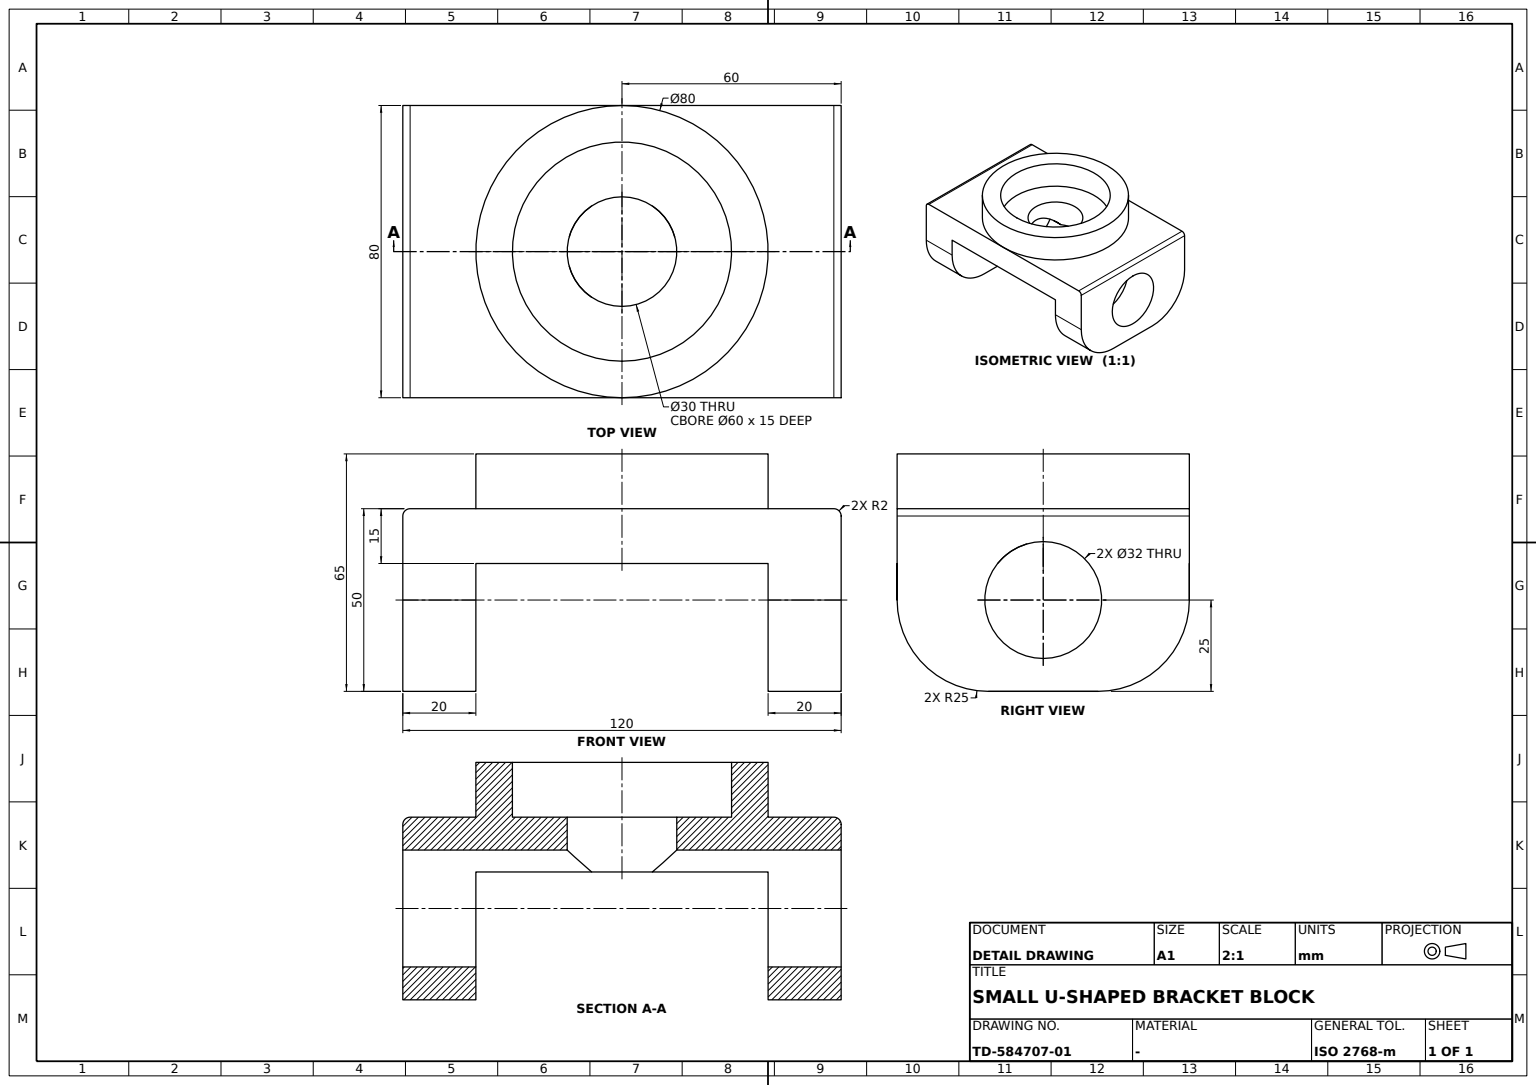
ISO-10303-21;
HEADER;
FILE_DESCRIPTION((''),'2;1');
FILE_NAME('','',(''),(''),'','','');
FILE_SCHEMA(('AUTOMOTIVE_DESIGN'));
ENDSEC;
DATA;
#1=APPLICATION_CONTEXT('');
#2=PRODUCT_CONTEXT('',#1,'mechanical');
#3=PRODUCT('','','',(#2));
#4=PRODUCT_DEFINITION_FORMATION('','',#3);
#5=PRODUCT_DEFINITION_CONTEXT('',#1,'design');
#6=PRODUCT_DEFINITION('','',#4,#5);
#7=PRODUCT_DEFINITION_SHAPE('','',#6);
#8=(LENGTH_UNIT()NAMED_UNIT(*)SI_UNIT(.MILLI.,.METRE.));
#9=(NAMED_UNIT(*)PLANE_ANGLE_UNIT()SI_UNIT($,.RADIAN.));
#10=(NAMED_UNIT(*)SI_UNIT($,.STERADIAN.)SOLID_ANGLE_UNIT());
#11=UNCERTAINTY_MEASURE_WITH_UNIT(LENGTH_MEASURE(0.005),#8,'distance_accuracy_value','');
#12=(GEOMETRIC_REPRESENTATION_CONTEXT(3)GLOBAL_UNCERTAINTY_ASSIGNED_CONTEXT((#11))GLOBAL_UNIT_ASSIGNED_CONTEXT((#8,#9,#10))REPRESENTATION_CONTEXT('',''));
#13=CARTESIAN_POINT('',(12.489996,40.,0.));
#14=VERTEX_POINT('',#13);
#15=CARTESIAN_POINT('',(40.,40.,0.));
#16=VERTEX_POINT('',#15);
#17=CARTESIAN_POINT('',(0.,40.,0.));
#18=DIRECTION('',(1.,0.,0.));
#19=VECTOR('',#18,1000.);
#20=LINE('',#17,#19);
#21=EDGE_CURVE('',#14,#16,#20,.T.);
#22=ORIENTED_EDGE('',*,*,#21,.T.);
#23=CARTESIAN_POINT('',(40.,-40.,0.));
#24=VERTEX_POINT('',#23);
#25=CARTESIAN_POINT('',(40.,0.,0.));
#26=DIRECTION('',(0.,1.,0.));
#27=VECTOR('',#26,1000.);
#28=LINE('',#25,#27);
#29=EDGE_CURVE('',#24,#16,#28,.T.);
#30=ORIENTED_EDGE('',*,*,#29,.F.);
#31=CARTESIAN_POINT('',(12.489996,-40.,0.));
#32=VERTEX_POINT('',#31);
#33=CARTESIAN_POINT('',(0.,-40.,0.));
#34=LINE('',#33,#19);
#35=EDGE_CURVE('',#32,#24,#34,.T.);
#36=ORIENTED_EDGE('',*,*,#35,.F.);
#37=CARTESIAN_POINT('',(12.489996,-8.306624,0.));
#38=VERTEX_POINT('',#37);
#39=LINE('',#31,#27);
#40=EDGE_CURVE('',#38,#32,#39,.F.);
#41=ORIENTED_EDGE('',*,*,#40,.F.);
#42=CARTESIAN_POINT('',(12.489996,8.306624,0.));
#43=VERTEX_POINT('',#42);
#44=CARTESIAN_POINT('',(0.,0.,0.));
#45=DIRECTION('',(0.,0.,-1.));
#46=DIRECTION('',(-1.,0.,0.));
#47=AXIS2_PLACEMENT_3D('',#44,#45,#46);
#48=CIRCLE('',#47,15.);
#49=EDGE_CURVE('',#38,#43,#48,.F.);
#50=ORIENTED_EDGE('',*,*,#49,.T.);
#51=LINE('',#42,#27);
#52=EDGE_CURVE('',#14,#43,#51,.F.);
#53=ORIENTED_EDGE('',*,*,#52,.F.);
#54=EDGE_LOOP('',(#22,#30,#36,#41,#50,#53));
#55=FACE_BOUND('',#54,.T.);
#56=AXIS2_PLACEMENT_3D('',#33,#45,#26);
#57=PLANE('',#56);
#58=ADVANCED_FACE('',(#55),#57,.T.);
#59=CARTESIAN_POINT('',(0.,-60.,-26.));
#60=VERTEX_POINT('',#59);
#61=CARTESIAN_POINT('',(0.,-60.,-10.));
#62=DIRECTION('',(0.,-1.,0.));
#63=AXIS2_PLACEMENT_3D('',#61,#62,#45);
#64=CIRCLE('',#63,16.);
#65=EDGE_CURVE('',#60,#60,#64,.T.);
#66=ORIENTED_EDGE('',*,*,#65,.F.);
#67=EDGE_LOOP('',(#66));
#68=FACE_BOUND('',#67,.T.);
#69=CARTESIAN_POINT('',(15.,-60.,-35.));
#70=VERTEX_POINT('',#69);
#71=CARTESIAN_POINT('',(40.,-60.,-10.));
#72=VERTEX_POINT('',#71);
#73=CARTESIAN_POINT('',(15.,-60.,-10.));
#74=AXIS2_PLACEMENT_3D('',#73,#62,#45);
#75=CIRCLE('',#74,25.);
#76=EDGE_CURVE('',#70,#72,#75,.T.);
#77=ORIENTED_EDGE('',*,*,#76,.T.);
#78=CARTESIAN_POINT('',(40.,-60.,13.));
#79=VERTEX_POINT('',#78);
#80=CARTESIAN_POINT('',(40.,-60.,0.));
#81=VECTOR('',#45,1000.);
#82=LINE('',#80,#81);
#83=EDGE_CURVE('',#79,#72,#82,.T.);
#84=ORIENTED_EDGE('',*,*,#83,.F.);
#85=CARTESIAN_POINT('',(-40.,-60.,13.));
#86=VERTEX_POINT('',#85);
#87=CARTESIAN_POINT('',(0.,-60.,13.));
#88=LINE('',#87,#19);
#89=EDGE_CURVE('',#86,#79,#88,.T.);
#90=ORIENTED_EDGE('',*,*,#89,.F.);
#91=CARTESIAN_POINT('',(-40.,-60.,-10.));
#92=VERTEX_POINT('',#91);
#93=CARTESIAN_POINT('',(-40.,-60.,0.));
#94=LINE('',#93,#81);
#95=EDGE_CURVE('',#86,#92,#94,.T.);
#96=ORIENTED_EDGE('',*,*,#95,.T.);
#97=CARTESIAN_POINT('',(-15.,-60.,-35.));
#98=VERTEX_POINT('',#97);
#99=CARTESIAN_POINT('',(-15.,-60.,-10.));
#100=AXIS2_PLACEMENT_3D('',#99,#62,#45);
#101=CIRCLE('',#100,25.);
#102=EDGE_CURVE('',#92,#98,#101,.T.);
#103=ORIENTED_EDGE('',*,*,#102,.T.);
#104=CARTESIAN_POINT('',(0.,-60.,-35.));
#105=LINE('',#104,#19);
#106=EDGE_CURVE('',#98,#70,#105,.T.);
#107=ORIENTED_EDGE('',*,*,#106,.T.);
#108=EDGE_LOOP('',(#77,#84,#90,#96,#103,#107));
#109=FACE_BOUND('',#108,.T.);
#110=CARTESIAN_POINT('',(0.,-60.,15.));
#111=AXIS2_PLACEMENT_3D('',#110,#62,#45);
#112=PLANE('',#111);
#113=ADVANCED_FACE('',(#68,#109),#112,.T.);
#114=ORIENTED_EDGE('',*,*,#35,.T.);
#115=CARTESIAN_POINT('',(40.,-40.,-10.));
#116=VERTEX_POINT('',#115);
#117=DIRECTION('',(0.,0.,1.));
#118=VECTOR('',#117,1000.);
#119=LINE('',#23,#118);
#120=EDGE_CURVE('',#116,#24,#119,.T.);
#121=ORIENTED_EDGE('',*,*,#120,.F.);
#122=CARTESIAN_POINT('',(15.,-40.,-35.));
#123=VERTEX_POINT('',#122);
#124=CARTESIAN_POINT('',(15.,-40.,-10.));
#125=AXIS2_PLACEMENT_3D('',#124,#26,#117);
#126=CIRCLE('',#125,25.);
#127=EDGE_CURVE('',#116,#123,#126,.T.);
#128=ORIENTED_EDGE('',*,*,#127,.T.);
#129=CARTESIAN_POINT('',(-15.,-40.,-35.));
#130=VERTEX_POINT('',#129);
#131=CARTESIAN_POINT('',(0.,-40.,-35.));
#132=LINE('',#131,#19);
#133=EDGE_CURVE('',#130,#123,#132,.T.);
#134=ORIENTED_EDGE('',*,*,#133,.F.);
#135=CARTESIAN_POINT('',(-40.,-40.,-10.));
#136=VERTEX_POINT('',#135);
#137=CARTESIAN_POINT('',(-15.,-40.,-10.));
#138=AXIS2_PLACEMENT_3D('',#137,#26,#117);
#139=CIRCLE('',#138,25.);
#140=EDGE_CURVE('',#130,#136,#139,.T.);
#141=ORIENTED_EDGE('',*,*,#140,.T.);
#142=CARTESIAN_POINT('',(-40.,-40.,0.));
#143=VERTEX_POINT('',#142);
#144=LINE('',#142,#118);
#145=EDGE_CURVE('',#136,#143,#144,.T.);
#146=ORIENTED_EDGE('',*,*,#145,.T.);
#147=CARTESIAN_POINT('',(-12.489996,-40.,0.));
#148=VERTEX_POINT('',#147);
#149=EDGE_CURVE('',#143,#148,#34,.T.);
#150=ORIENTED_EDGE('',*,*,#149,.T.);
#151=CARTESIAN_POINT('',(0.,-40.,-10.));
#152=AXIS2_PLACEMENT_3D('',#151,#26,#117);
#153=CIRCLE('',#152,16.);
#154=EDGE_CURVE('',#32,#148,#153,.T.);
#155=ORIENTED_EDGE('',*,*,#154,.F.);
#156=EDGE_LOOP('',(#114,#121,#128,#134,#141,#146,#150,#155));
#157=FACE_BOUND('',#156,.T.);
#158=AXIS2_PLACEMENT_3D('',#131,#26,#117);
#159=PLANE('',#158);
#160=ADVANCED_FACE('',(#157),#159,.T.);
#161=CARTESIAN_POINT('',(40.,60.,-10.));
#162=VERTEX_POINT('',#161);
#163=CARTESIAN_POINT('',(40.,60.,13.));
#164=VERTEX_POINT('',#163);
#165=CARTESIAN_POINT('',(40.,60.,0.));
#166=LINE('',#165,#118);
#167=EDGE_CURVE('',#162,#164,#166,.T.);
#168=ORIENTED_EDGE('',*,*,#167,.F.);
#169=CARTESIAN_POINT('',(15.,60.,-35.));
#170=VERTEX_POINT('',#169);
#171=CARTESIAN_POINT('',(15.,60.,-10.));
#172=AXIS2_PLACEMENT_3D('',#171,#26,#117);
#173=CIRCLE('',#172,25.);
#174=EDGE_CURVE('',#162,#170,#173,.T.);
#175=ORIENTED_EDGE('',*,*,#174,.T.);
#176=CARTESIAN_POINT('',(-15.,60.,-35.));
#177=VERTEX_POINT('',#176);
#178=CARTESIAN_POINT('',(0.,60.,-35.));
#179=LINE('',#178,#19);
#180=EDGE_CURVE('',#177,#170,#179,.T.);
#181=ORIENTED_EDGE('',*,*,#180,.F.);
#182=CARTESIAN_POINT('',(-40.,60.,-10.));
#183=VERTEX_POINT('',#182);
#184=CARTESIAN_POINT('',(-15.,60.,-10.));
#185=AXIS2_PLACEMENT_3D('',#184,#26,#117);
#186=CIRCLE('',#185,25.);
#187=EDGE_CURVE('',#177,#183,#186,.T.);
#188=ORIENTED_EDGE('',*,*,#187,.T.);
#189=CARTESIAN_POINT('',(-40.,60.,13.));
#190=VERTEX_POINT('',#189);
#191=CARTESIAN_POINT('',(-40.,60.,0.));
#192=LINE('',#191,#118);
#193=EDGE_CURVE('',#183,#190,#192,.T.);
#194=ORIENTED_EDGE('',*,*,#193,.T.);
#195=CARTESIAN_POINT('',(0.,60.,13.));
#196=LINE('',#195,#19);
#197=EDGE_CURVE('',#190,#164,#196,.T.);
#198=ORIENTED_EDGE('',*,*,#197,.T.);
#199=EDGE_LOOP('',(#168,#175,#181,#188,#194,#198));
#200=FACE_BOUND('',#199,.T.);
#201=CARTESIAN_POINT('',(0.,60.,6.));
#202=VERTEX_POINT('',#201);
#203=CARTESIAN_POINT('',(0.,60.,-10.));
#204=AXIS2_PLACEMENT_3D('',#203,#26,#117);
#205=CIRCLE('',#204,16.);
#206=EDGE_CURVE('',#202,#202,#205,.T.);
#207=ORIENTED_EDGE('',*,*,#206,.F.);
#208=EDGE_LOOP('',(#207));
#209=FACE_BOUND('',#208,.T.);
#210=AXIS2_PLACEMENT_3D('',#178,#26,#117);
#211=PLANE('',#210);
#212=ADVANCED_FACE('',(#200,#209),#211,.T.);
#213=CARTESIAN_POINT('',(40.,0.,15.));
#214=VERTEX_POINT('',#213);
#215=CARTESIAN_POINT('',(-40.,0.,15.));
#216=VERTEX_POINT('',#215);
#217=CARTESIAN_POINT('',(0.,0.,15.));
#218=AXIS2_PLACEMENT_3D('',#217,#117,#18);
#219=CIRCLE('',#218,40.);
#220=EDGE_CURVE('',#214,#216,#219,.T.);
#221=ORIENTED_EDGE('',*,*,#220,.T.);
#222=EDGE_CURVE('',#216,#214,#219,.T.);
#223=ORIENTED_EDGE('',*,*,#222,.T.);
#224=EDGE_LOOP('',(#221,#223));
#225=FACE_BOUND('',#224,.T.);
#226=CARTESIAN_POINT('',(40.,0.,30.));
#227=VERTEX_POINT('',#226);
#228=CARTESIAN_POINT('',(0.,0.,30.));
#229=AXIS2_PLACEMENT_3D('',#228,#117,#18);
#230=CIRCLE('',#229,40.);
#231=EDGE_CURVE('',#227,#227,#230,.T.);
#232=ORIENTED_EDGE('',*,*,#231,.F.);
#233=EDGE_LOOP('',(#232));
#234=FACE_BOUND('',#233,.T.);
#235=CARTESIAN_POINT('',(0.,0.,22.5));
#236=AXIS2_PLACEMENT_3D('',#235,#117,#18);
#237=CYLINDRICAL_SURFACE('',#236,40.);
#238=ADVANCED_FACE('',(#225,#234),#237,.T.);
#239=CARTESIAN_POINT('',(-40.,40.,-10.));
#240=VERTEX_POINT('',#239);
#241=CARTESIAN_POINT('',(-40.,0.,-10.));
#242=LINE('',#241,#27);
#243=EDGE_CURVE('',#240,#183,#242,.T.);
#244=ORIENTED_EDGE('',*,*,#243,.T.);
#245=ORIENTED_EDGE('',*,*,#187,.F.);
#246=CARTESIAN_POINT('',(-15.,40.,-35.));
#247=VERTEX_POINT('',#246);
#248=CARTESIAN_POINT('',(-15.,0.,-35.));
#249=LINE('',#248,#27);
#250=EDGE_CURVE('',#247,#177,#249,.T.);
#251=ORIENTED_EDGE('',*,*,#250,.F.);
#252=CARTESIAN_POINT('',(-15.,40.,-10.));
#253=AXIS2_PLACEMENT_3D('',#252,#62,#45);
#254=CIRCLE('',#253,25.);
#255=EDGE_CURVE('',#240,#247,#254,.T.);
#256=ORIENTED_EDGE('',*,*,#255,.F.);
#257=EDGE_LOOP('',(#244,#245,#251,#256));
#258=FACE_BOUND('',#257,.T.);
#259=CARTESIAN_POINT('',(-15.,0.,-10.));
#260=AXIS2_PLACEMENT_3D('',#259,#26,#46);
#261=CYLINDRICAL_SURFACE('',#260,25.);
#262=ADVANCED_FACE('',(#258),#261,.T.);
#263=EDGE_CURVE('',#98,#130,#249,.T.);
#264=ORIENTED_EDGE('',*,*,#263,.F.);
#265=ORIENTED_EDGE('',*,*,#102,.F.);
#266=EDGE_CURVE('',#92,#136,#242,.T.);
#267=ORIENTED_EDGE('',*,*,#266,.T.);
#268=ORIENTED_EDGE('',*,*,#140,.F.);
#269=EDGE_LOOP('',(#264,#265,#267,#268));
#270=FACE_BOUND('',#269,.T.);
#271=ADVANCED_FACE('',(#270),#261,.T.);
#272=ORIENTED_EDGE('',*,*,#29,.T.);
#273=CARTESIAN_POINT('',(40.,40.,-10.));
#274=VERTEX_POINT('',#273);
#275=LINE('',#15,#81);
#276=EDGE_CURVE('',#16,#274,#275,.T.);
#277=ORIENTED_EDGE('',*,*,#276,.T.);
#278=CARTESIAN_POINT('',(40.,0.,-10.));
#279=LINE('',#278,#27);
#280=EDGE_CURVE('',#274,#162,#279,.T.);
#281=ORIENTED_EDGE('',*,*,#280,.T.);
#282=ORIENTED_EDGE('',*,*,#167,.T.);
#283=CARTESIAN_POINT('',(40.,58.,15.));
#284=VERTEX_POINT('',#283);
#285=CARTESIAN_POINT('',(40.,58.,13.));
#286=AXIS2_PLACEMENT_3D('',#285,#18,#45);
#287=CIRCLE('',#286,2.);
#288=EDGE_CURVE('',#164,#284,#287,.T.);
#289=ORIENTED_EDGE('',*,*,#288,.T.);
#290=VECTOR('',#62,1000.);
#291=LINE('',#213,#290);
#292=EDGE_CURVE('',#284,#214,#291,.T.);
#293=ORIENTED_EDGE('',*,*,#292,.T.);
#294=CARTESIAN_POINT('',(40.,-58.,15.));
#295=VERTEX_POINT('',#294);
#296=EDGE_CURVE('',#214,#295,#291,.T.);
#297=ORIENTED_EDGE('',*,*,#296,.T.);
#298=CARTESIAN_POINT('',(40.,-58.,13.));
#299=AXIS2_PLACEMENT_3D('',#298,#18,#45);
#300=CIRCLE('',#299,2.);
#301=EDGE_CURVE('',#295,#79,#300,.T.);
#302=ORIENTED_EDGE('',*,*,#301,.T.);
#303=ORIENTED_EDGE('',*,*,#83,.T.);
#304=EDGE_CURVE('',#72,#116,#279,.T.);
#305=ORIENTED_EDGE('',*,*,#304,.T.);
#306=ORIENTED_EDGE('',*,*,#120,.T.);
#307=EDGE_LOOP('',(#272,#277,#281,#282,#289,#293,#297,#302,#303,#305,#306));
#308=FACE_BOUND('',#307,.T.);
#309=AXIS2_PLACEMENT_3D('',#25,#18,#26);
#310=PLANE('',#309);
#311=ADVANCED_FACE('',(#308),#310,.T.);
#312=ORIENTED_EDGE('',*,*,#220,.F.);
#313=ORIENTED_EDGE('',*,*,#292,.F.);
#314=CARTESIAN_POINT('',(-40.,58.,15.));
#315=VERTEX_POINT('',#314);
#316=CARTESIAN_POINT('',(0.,58.,15.));
#317=LINE('',#316,#19);
#318=EDGE_CURVE('',#315,#284,#317,.T.);
#319=ORIENTED_EDGE('',*,*,#318,.F.);
#320=LINE('',#215,#290);
#321=EDGE_CURVE('',#315,#216,#320,.T.);
#322=ORIENTED_EDGE('',*,*,#321,.T.);
#323=EDGE_LOOP('',(#312,#313,#319,#322));
#324=FACE_BOUND('',#323,.T.);
#325=CARTESIAN_POINT('',(0.,60.,15.));
#326=AXIS2_PLACEMENT_3D('',#325,#117,#62);
#327=PLANE('',#326);
#328=ADVANCED_FACE('',(#324),#327,.T.);
#329=ORIENTED_EDGE('',*,*,#231,.T.);
#330=EDGE_LOOP('',(#329));
#331=FACE_BOUND('',#330,.T.);
#332=CARTESIAN_POINT('',(30.,0.,30.));
#333=VERTEX_POINT('',#332);
#334=CIRCLE('',#229,30.);
#335=EDGE_CURVE('',#333,#333,#334,.T.);
#336=ORIENTED_EDGE('',*,*,#335,.F.);
#337=EDGE_LOOP('',(#336));
#338=FACE_BOUND('',#337,.T.);
#339=PLANE('',#229);
#340=ADVANCED_FACE('',(#331,#338),#339,.T.);
#341=CARTESIAN_POINT('',(-40.,-58.,15.));
#342=VERTEX_POINT('',#341);
#343=CARTESIAN_POINT('',(-40.,-58.,13.));
#344=AXIS2_PLACEMENT_3D('',#343,#18,#45);
#345=CIRCLE('',#344,2.);
#346=EDGE_CURVE('',#342,#86,#345,.T.);
#347=ORIENTED_EDGE('',*,*,#346,.F.);
#348=EDGE_CURVE('',#216,#342,#320,.T.);
#349=ORIENTED_EDGE('',*,*,#348,.F.);
#350=ORIENTED_EDGE('',*,*,#321,.F.);
#351=CARTESIAN_POINT('',(-40.,58.,13.));
#352=AXIS2_PLACEMENT_3D('',#351,#18,#45);
#353=CIRCLE('',#352,2.);
#354=EDGE_CURVE('',#190,#315,#353,.T.);
#355=ORIENTED_EDGE('',*,*,#354,.F.);
#356=ORIENTED_EDGE('',*,*,#193,.F.);
#357=ORIENTED_EDGE('',*,*,#243,.F.);
#358=CARTESIAN_POINT('',(-40.,40.,0.));
#359=VERTEX_POINT('',#358);
#360=LINE('',#358,#81);
#361=EDGE_CURVE('',#359,#240,#360,.T.);
#362=ORIENTED_EDGE('',*,*,#361,.F.);
#363=CARTESIAN_POINT('',(-40.,0.,0.));
#364=LINE('',#363,#27);
#365=EDGE_CURVE('',#143,#359,#364,.T.);
#366=ORIENTED_EDGE('',*,*,#365,.F.);
#367=ORIENTED_EDGE('',*,*,#145,.F.);
#368=ORIENTED_EDGE('',*,*,#266,.F.);
#369=ORIENTED_EDGE('',*,*,#95,.F.);
#370=EDGE_LOOP('',(#347,#349,#350,#355,#356,#357,#362,#366,#367,#368,#369));
#371=FACE_BOUND('',#370,.T.);
#372=AXIS2_PLACEMENT_3D('',#363,#18,#26);
#373=PLANE('',#372);
#374=ADVANCED_FACE('',(#371),#373,.F.);
#375=ORIENTED_EDGE('',*,*,#301,.F.);
#376=CARTESIAN_POINT('',(0.,-58.,15.));
#377=LINE('',#376,#19);
#378=EDGE_CURVE('',#342,#295,#377,.T.);
#379=ORIENTED_EDGE('',*,*,#378,.F.);
#380=ORIENTED_EDGE('',*,*,#346,.T.);
#381=ORIENTED_EDGE('',*,*,#89,.T.);
#382=EDGE_LOOP('',(#375,#379,#380,#381));
#383=FACE_BOUND('',#382,.T.);
#384=CARTESIAN_POINT('',(0.,-58.,13.));
#385=AXIS2_PLACEMENT_3D('',#384,#18,#62);
#386=CYLINDRICAL_SURFACE('',#385,2.);
#387=ADVANCED_FACE('',(#383),#386,.T.);
#388=CARTESIAN_POINT('',(30.,0.,15.));
#389=VERTEX_POINT('',#388);
#390=CIRCLE('',#218,30.);
#391=EDGE_CURVE('',#389,#389,#390,.T.);
#392=ORIENTED_EDGE('',*,*,#391,.T.);
#393=EDGE_LOOP('',(#392));
#394=FACE_BOUND('',#393,.T.);
#395=CARTESIAN_POINT('',(15.,0.,15.));
#396=VERTEX_POINT('',#395);
#397=CIRCLE('',#218,15.);
#398=EDGE_CURVE('',#396,#396,#397,.T.);
#399=ORIENTED_EDGE('',*,*,#398,.F.);
#400=EDGE_LOOP('',(#399));
#401=FACE_BOUND('',#400,.T.);
#402=ADVANCED_FACE('',(#394,#401),#327,.T.);
#403=CARTESIAN_POINT('',(15.,40.,-35.));
#404=VERTEX_POINT('',#403);
#405=CARTESIAN_POINT('',(15.,0.,-35.));
#406=LINE('',#405,#27);
#407=EDGE_CURVE('',#404,#170,#406,.T.);
#408=ORIENTED_EDGE('',*,*,#407,.T.);
#409=ORIENTED_EDGE('',*,*,#174,.F.);
#410=ORIENTED_EDGE('',*,*,#280,.F.);
#411=CARTESIAN_POINT('',(15.,40.,-10.));
#412=AXIS2_PLACEMENT_3D('',#411,#62,#45);
#413=CIRCLE('',#412,25.);
#414=EDGE_CURVE('',#404,#274,#413,.T.);
#415=ORIENTED_EDGE('',*,*,#414,.F.);
#416=EDGE_LOOP('',(#408,#409,#410,#415));
#417=FACE_BOUND('',#416,.T.);
#418=CARTESIAN_POINT('',(15.,0.,-10.));
#419=AXIS2_PLACEMENT_3D('',#418,#26,#45);
#420=CYLINDRICAL_SURFACE('',#419,25.);
#421=ADVANCED_FACE('',(#417),#420,.T.);
#422=ORIENTED_EDGE('',*,*,#318,.T.);
#423=ORIENTED_EDGE('',*,*,#288,.F.);
#424=ORIENTED_EDGE('',*,*,#197,.F.);
#425=ORIENTED_EDGE('',*,*,#354,.T.);
#426=EDGE_LOOP('',(#422,#423,#424,#425));
#427=FACE_BOUND('',#426,.T.);
#428=CARTESIAN_POINT('',(0.,58.,13.));
#429=AXIS2_PLACEMENT_3D('',#428,#18,#117);
#430=CYLINDRICAL_SURFACE('',#429,2.);
#431=ADVANCED_FACE('',(#427),#430,.T.);
#432=CARTESIAN_POINT('',(-12.489996,-8.306624,0.));
#433=VERTEX_POINT('',#432);
#434=CARTESIAN_POINT('',(-11.254734,-10.163987,1.542842));
#435=CARTESIAN_POINT('',(-8.780673,-12.594948,3.761634));
#436=CARTESIAN_POINT('',(-4.057516,-14.624106,5.64612));
#437=CARTESIAN_POINT('',(-0.009777,-15.18652,6.1756));
#438=CARTESIAN_POINT('',(4.036962,-14.629796,5.65146));
#439=CARTESIAN_POINT('',(8.769467,-12.604832,3.770687));
#440=CARTESIAN_POINT('',(11.253492,-10.165855,1.544393));
#441=B_SPLINE_CURVE_WITH_KNOTS('',3,(#432,#434,#435,#436,#437,#438,#439,#440,#37),.UNSPECIFIED.,.F.,.F.,(4,1,1,1,1,1,4),(0.,0.008039872,0.012059808,0.016079745,0.020099681,0.024119617,0.032159489),.UNSPECIFIED.);
#442=EDGE_CURVE('',#433,#38,#441,.T.);
#443=ORIENTED_EDGE('',*,*,#442,.T.);
#444=ORIENTED_EDGE('',*,*,#40,.T.);
#445=ORIENTED_EDGE('',*,*,#154,.T.);
#446=LINE('',#147,#27);
#447=EDGE_CURVE('',#148,#433,#446,.T.);
#448=ORIENTED_EDGE('',*,*,#447,.T.);
#449=EDGE_LOOP('',(#443,#444,#445,#448));
#450=FACE_BOUND('',#449,.T.);
#451=ORIENTED_EDGE('',*,*,#65,.T.);
#452=EDGE_LOOP('',(#451));
#453=FACE_BOUND('',#452,.T.);
#454=CARTESIAN_POINT('',(0.,-0.66,-10.));
#455=AXIS2_PLACEMENT_3D('',#454,#26,#46);
#456=CYLINDRICAL_SURFACE('',#455,16.);
#457=ADVANCED_FACE('',(#450,#453),#456,.F.);
#458=ORIENTED_EDGE('',*,*,#206,.T.);
#459=EDGE_LOOP('',(#458));
#460=FACE_BOUND('',#459,.T.);
#461=CARTESIAN_POINT('',(-12.489996,40.,0.));
#462=VERTEX_POINT('',#461);
#463=CARTESIAN_POINT('',(0.,40.,-10.));
#464=AXIS2_PLACEMENT_3D('',#463,#62,#45);
#465=CIRCLE('',#464,16.);
#466=EDGE_CURVE('',#462,#14,#465,.T.);
#467=ORIENTED_EDGE('',*,*,#466,.T.);
#468=ORIENTED_EDGE('',*,*,#52,.T.);
#469=CARTESIAN_POINT('',(-12.489996,8.306624,0.));
#470=VERTEX_POINT('',#469);
#471=CARTESIAN_POINT('',(11.254734,10.163987,1.542842));
#472=CARTESIAN_POINT('',(8.780673,12.594948,3.761634));
#473=CARTESIAN_POINT('',(4.057516,14.624106,5.64612));
#474=CARTESIAN_POINT('',(0.009777,15.18652,6.1756));
#475=CARTESIAN_POINT('',(-4.036962,14.629796,5.65146));
#476=CARTESIAN_POINT('',(-8.769467,12.604832,3.770687));
#477=CARTESIAN_POINT('',(-11.253492,10.165855,1.544393));
#478=B_SPLINE_CURVE_WITH_KNOTS('',3,(#42,#471,#472,#473,#474,#475,#476,#477,#469),.UNSPECIFIED.,.F.,.F.,(4,1,1,1,1,1,4),(0.,0.008039872,0.012059808,0.016079745,0.020099681,0.024119617,0.032159489),.UNSPECIFIED.);
#479=EDGE_CURVE('',#43,#470,#478,.T.);
#480=ORIENTED_EDGE('',*,*,#479,.T.);
#481=LINE('',#469,#27);
#482=EDGE_CURVE('',#470,#462,#481,.T.);
#483=ORIENTED_EDGE('',*,*,#482,.T.);
#484=EDGE_LOOP('',(#467,#468,#480,#483));
#485=FACE_BOUND('',#484,.T.);
#486=ADVANCED_FACE('',(#460,#485),#456,.F.);
#487=ORIENTED_EDGE('',*,*,#378,.T.);
#488=ORIENTED_EDGE('',*,*,#296,.F.);
#489=ORIENTED_EDGE('',*,*,#222,.F.);
#490=ORIENTED_EDGE('',*,*,#348,.T.);
#491=EDGE_LOOP('',(#487,#488,#489,#490));
#492=FACE_BOUND('',#491,.T.);
#493=ADVANCED_FACE('',(#492),#327,.T.);
#494=ORIENTED_EDGE('',*,*,#447,.F.);
#495=ORIENTED_EDGE('',*,*,#149,.F.);
#496=ORIENTED_EDGE('',*,*,#365,.T.);
#497=EDGE_CURVE('',#359,#462,#20,.T.);
#498=ORIENTED_EDGE('',*,*,#497,.T.);
#499=ORIENTED_EDGE('',*,*,#482,.F.);
#500=EDGE_CURVE('',#470,#433,#48,.F.);
#501=ORIENTED_EDGE('',*,*,#500,.T.);
#502=EDGE_LOOP('',(#494,#495,#496,#498,#499,#501));
#503=FACE_BOUND('',#502,.T.);
#504=ADVANCED_FACE('',(#503),#57,.T.);
#505=EDGE_CURVE('',#70,#123,#406,.T.);
#506=ORIENTED_EDGE('',*,*,#505,.F.);
#507=ORIENTED_EDGE('',*,*,#106,.F.);
#508=ORIENTED_EDGE('',*,*,#263,.T.);
#509=ORIENTED_EDGE('',*,*,#133,.T.);
#510=EDGE_LOOP('',(#506,#507,#508,#509));
#511=FACE_BOUND('',#510,.T.);
#512=CARTESIAN_POINT('',(0.,40.,-35.));
#513=AXIS2_PLACEMENT_3D('',#512,#45,#26);
#514=PLANE('',#513);
#515=ADVANCED_FACE('',(#511),#514,.T.);
#516=ORIENTED_EDGE('',*,*,#500,.F.);
#517=ORIENTED_EDGE('',*,*,#479,.F.);
#518=ORIENTED_EDGE('',*,*,#49,.F.);
#519=ORIENTED_EDGE('',*,*,#442,.F.);
#520=EDGE_LOOP('',(#516,#517,#518,#519));
#521=FACE_BOUND('',#520,.T.);
#522=ORIENTED_EDGE('',*,*,#398,.T.);
#523=EDGE_LOOP('',(#522));
#524=FACE_BOUND('',#523,.T.);
#525=CARTESIAN_POINT('',(0.,0.,7.5));
#526=AXIS2_PLACEMENT_3D('',#525,#117,#18);
#527=CYLINDRICAL_SURFACE('',#526,15.);
#528=ADVANCED_FACE('',(#521,#524),#527,.F.);
#529=ORIENTED_EDGE('',*,*,#276,.F.);
#530=ORIENTED_EDGE('',*,*,#21,.F.);
#531=ORIENTED_EDGE('',*,*,#466,.F.);
#532=ORIENTED_EDGE('',*,*,#497,.F.);
#533=ORIENTED_EDGE('',*,*,#361,.T.);
#534=ORIENTED_EDGE('',*,*,#255,.T.);
#535=LINE('',#512,#19);
#536=EDGE_CURVE('',#247,#404,#535,.T.);
#537=ORIENTED_EDGE('',*,*,#536,.T.);
#538=ORIENTED_EDGE('',*,*,#414,.T.);
#539=EDGE_LOOP('',(#529,#530,#531,#532,#533,#534,#537,#538));
#540=FACE_BOUND('',#539,.T.);
#541=AXIS2_PLACEMENT_3D('',#17,#62,#45);
#542=PLANE('',#541);
#543=ADVANCED_FACE('',(#540),#542,.T.);
#544=ORIENTED_EDGE('',*,*,#391,.F.);
#545=EDGE_LOOP('',(#544));
#546=FACE_BOUND('',#545,.T.);
#547=ORIENTED_EDGE('',*,*,#335,.T.);
#548=EDGE_LOOP('',(#547));
#549=FACE_BOUND('',#548,.T.);
#550=CYLINDRICAL_SURFACE('',#236,30.);
#551=ADVANCED_FACE('',(#546,#549),#550,.F.);
#552=ORIENTED_EDGE('',*,*,#407,.F.);
#553=ORIENTED_EDGE('',*,*,#536,.F.);
#554=ORIENTED_EDGE('',*,*,#250,.T.);
#555=ORIENTED_EDGE('',*,*,#180,.T.);
#556=EDGE_LOOP('',(#552,#553,#554,#555));
#557=FACE_BOUND('',#556,.T.);
#558=ADVANCED_FACE('',(#557),#514,.T.);
#559=ORIENTED_EDGE('',*,*,#127,.F.);
#560=ORIENTED_EDGE('',*,*,#304,.F.);
#561=ORIENTED_EDGE('',*,*,#76,.F.);
#562=ORIENTED_EDGE('',*,*,#505,.T.);
#563=EDGE_LOOP('',(#559,#560,#561,#562));
#564=FACE_BOUND('',#563,.T.);
#565=ADVANCED_FACE('',(#564),#420,.T.);
#566=CLOSED_SHELL('',(#58,#113,#160,#212,#238,#262,#271,#311,#328,#340,#374,#387,#402,#421,#431,#457,#486,#493,#504,#515,#528,#543,#551,#558,#565));
#567=MANIFOLD_SOLID_BREP('',#566);
#568=ADVANCED_BREP_SHAPE_REPRESENTATION('',(#567),#12);
#569=SHAPE_DEFINITION_REPRESENTATION(#7,#568);
ENDSEC;
END-ISO-10303-21;
